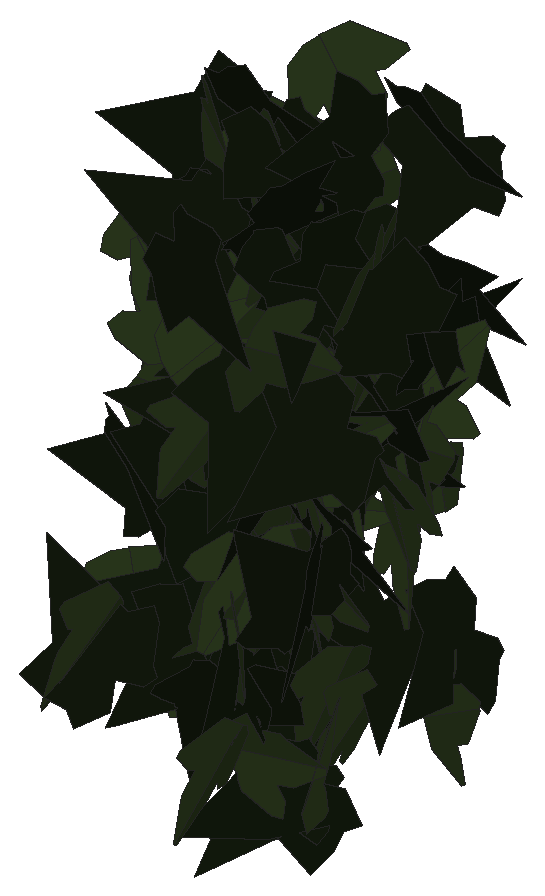
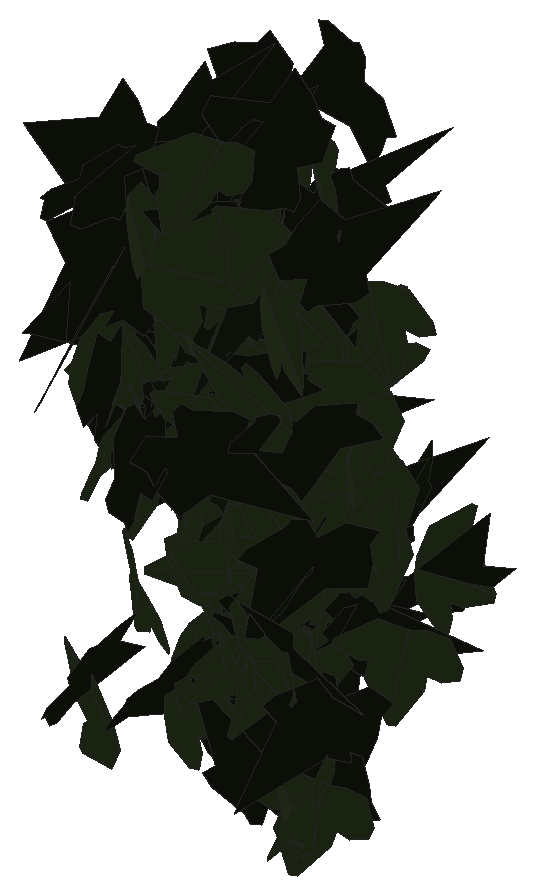
# SketchUp Ruby script. Lengths in inches.
U = 1.inch
M = Sketchup.active_model
def pt(a) = Geom::Point3d.new(a.map { |v| v * U })
def face(e, loops, mat)
  f = e.add_face(loops[0].map { |a| pt(a) })
  loops[1..].each { |l| e.add_face(l.map { |a| pt(a) }).erase! }
  f.material = f.back_material = mat if mat
  f
end
# faces: each face lists its corners as indices into pts; further lists are holes
def faces(e, pts, list, mat = nil) = list.each { |f| face(e, (f[0].is_a?(Array) ? f : [f]).map { |l| l.map { |i| pts[i] } }, mat) }
# xy, xz, yz: faces in a plane at the given z, y or x. An outline is a flat list of corners, or four numbers for a rectangle; further outlines are holes
def ring(l) = l.size == 4 ? [[l[0], l[1]], [l[2], l[1]], [l[2], l[3]], [l[0], l[3]]] : l.each_slice(2).to_a
def flat(e, list, mat, &to3) = list.each { |f| face(e, (f[0].is_a?(Array) ? f : [f]).map { |l| ring(l).map { |u, v| to3.(u, v) } }, mat) }
def xy(e, z, list, mat = nil) = flat(e, list, mat) { |x, y| [x, y, z] }
def xz(e, y, list, mat = nil) = flat(e, list, mat) { |x, z| [x, y, z] }
def yz(e, x, list, mat = nil) = flat(e, list, mat) { |y, z| [x, y, z] }
def lines(e, pts, list) = list.each { |a, b| e.add_line(pt(pts[a]), pt(pts[b])) }
# prism: a flat outline (further loops are holes) pulled along v
def prism(e, loops, v, mat = nil)
  f = face(e, loops, mat); d = Geom::Vector3d.new(v.map { |x| x * U })
  f.pushpull(f.normal.samedirection?(d) ? d.length : -d.length)
end
def box(e, o, s, mat = nil) = prism(e, [[o, [o[0] + s[0], o[1], o[2]], [o[0] + s[0], o[1] + s[1], o[2]], [o[0], o[1] + s[1], o[2]]]], [0, 0, s[2]], mat)
def at(x, y, z, deg = 0) = Geom::Transformation.translation(pt([x, y, z])) * Geom::Transformation.rotation(ORIGIN, Z_AXIS, deg.degrees)
def axes(o, x, y, z) = Geom::Transformation.new([*x, 0, *y, 0, *z, 0, *pt(o).to_a, 1])
def part(name) = M.definitions.add(name)
# library, detail: a bought-in or finely detailed component or shape, given as its bounding box
def library(name, o, s) = part(name).tap { |d| box(d.entities, o, s) }
def detail(e, o, s) = box(e.add_group.entities, o, s)
def put(e, d, t, mat = nil) = e.add_instance(d, t).tap { |i| i.material = mat if mat }
def group(e, t, mat = nil) = e.add_group.tap { |g| g.transformation = t; g.material = mat if mat }.entities
root = M.entities
M.materials.add("efeu1").color = [18, 25, 13]
M.materials.add("efeu2").color = [43, 57, 29]
c1 = part("ivyleaf_10")
p = [[0,0.5,-0.03],[-0.0625,2.02,-0.43],[-0.19,2.01,-0.46],[-0.54,1.05,-0.29],[-0.52,0.625,-0.18],[-0.83,0.76,-0.28],
  [-1.16,0.64,-0.33],[-1.15,0.33,-0.24],[-0.77,-0.39,0.02],[-0.3,-0.51,0.16],[0.04,-0.48,0.23],[-0.02,2.01,-0.4375],
  [-0.06,2.01,-0.43],[0.04,-0.49,0.23],[0.67,-0.49,0.14],[1.38,0.36,-0.2],[1.375,0.51,-0.24],[0.81,0.65,-0.19],
  [0.62,0.59,-0.15],[0.6,1.09,-0.28],[0.5,1.23,-0.31]]
faces(c1.entities,p,[[0,1,2,3,4,5,6,7,8,9,10],[11,12,0,13,14,15,16,17,18,19,20]],"efeu2")
c2 = part("ivyleaf_9")
p = [[1.54,2.16,1.25],[1.36,2.04,1.19],[-0.21,0.99,0.68],[-0.71,1.11,0.82],[-0.85,0.86,0.67],[-0.8,0.17,0.21],
  [-0.9,-0.01,0.1],[-0.67,-0.16,-0.02],[-0.08,-0.08,-0.05],[-0.03,-0.6,-0.4],[0.65,-0.88,-0.66],[0.83,-0.6,-0.49],
  [1.29,-0.42,-0.43],[1.8125,-0.07,-0.26],[1.21,0.44,0.15]]
faces(c2.entities,p,[[0,1,2,3,4,5,6,7,8,9,10,11,12,13,14]],"efeu1")
put(root,c1,axes([28.53,222.35,208.63],[0.41303,0.25945,0.10997],[0.09046,0.06274,-0.48773],[-0.26688,0.42279,0.00489]))
put(root,c2,axes([28.9,223.32,212.99],[-0.05885,-0.0343,0.49534],[-0.41168,-0.2755,-0.06799],[0.27759,-0.41584,0.00418]))
put(root,c1,axes([28.39,223.03,209.91],[-0.23609,-0.00713,0.4407],[0.44021,-0.02857,0.23536],[0.02183,0.49913,0.01977]))
put(root,c2,axes([28.59,223.36,208.42],[0.0425,-0.18384,-0.46303],[-0.03263,0.46269,-0.1867],[0.49712,0.04609,0.02733]))
put(root,c2,axes([28.59,223.66,210.3125],[-0.02142,-0.30956,-0.39207],[0.02032,0.39156,-0.31027],[0.49913,-0.02922,-0.00419]))
put(root,c1,axes([28.71,223.6,207.47],[-0.0357,0.46092,-0.19048],[0.01728,-0.18971,-0.46229],[-0.49842,-0.03959,-0.00238]))
put(root,c2,axes([28.98,222.45,209.85],[-0.08439,-0.03512,0.49157],[-0.37944,-0.31362,-0.08755],[0.31448,-0.38783,0.02628]))
put(root,c1,axes([28.68,222.5,209.8125],[-0.06336,-0.09851,-0.48609],[0.23876,0.42346,-0.11694],[0.43472,-0.24693,-0.00662]))
put(root,c1,axes([28.63,222.67,210.59],[-0.25398,-0.13068,-0.41039],[0.35505,0.20615,-0.28538],[0.24379,-0.43638,-0.01192]))
put(root,c1,axes([28.82,222.47,212.39],[0.4959,0.06356,-0.00651],[-0.00646,-0.00079,-0.49996],[-0.06356,0.49594,0.00004]))
put(root,c2,axes([28.6,222.36,209.89],[0.1419,-0.3425,0.3355],[0.12882,-0.30979,-0.37073],[0.46181,0.19164,0.00032]))
put(root,c1,axes([28.75,223.375,207.3125],[0.39362,0.258,0.16882],[0.14244,0.09063,-0.47063],[-0.27345,0.4186,-0.00215]))
put(root,c2,axes([28.84,223.625,211.5],[-0.19523,-0.4222,-0.18339],[0.08014,0.16498,-0.46514],[0.45328,-0.21101,0.00326]))
put(root,c1,axes([29.08,223.88,209.38],[0.0284,0.14804,0.47674],[-0.08611,-0.4689,0.15074],[0.49171,-0.09066,-0.00114]))
put(root,c1,axes([29.11,222.83,210.23],[-0.2734,-0.39024,0.15154],[-0.07857,-0.12995,-0.47638],[0.41119,-0.2843,0.00974]))
put(root,c1,axes([29.09,222.35,211.47],[0.21956,0.42607,0.14233],[-0.07184,-0.12307,0.47926],[0.44343,-0.23091,0.00717]))
put(root,c1,axes([28.76,222.89,210.82],[0.00696,-0.07393,0.49445],[0.38963,-0.30906,-0.0517],[0.31328,0.38603,0.05331]))
put(root,c2,axes([29.42,222.25,208.53],[-0.22412,-0.16527,-0.41528],[-0.29701,-0.29209,0.27653],[-0.334,0.37063,0.03275]))
put(root,c1,axes([29.04,221.26,208.84],[0.06989,-0.30517,0.38986],[0.06842,-0.38399,-0.31284],[0.49034,0.09708,-0.01191]))
put(root,c2,axes([29.26,221.14,208.36],[-0.3228,-0.36528,0.11122],[0.07397,0.08305,0.48747],[-0.3746,0.33117,0.00042]))
put(root,c2,axes([29.38,223.83,209.23],[-0.47607,0.06129,0.14],[-0.1384,0.02143,-0.47999],[-0.06483,-0.49577,-0.00344]))
put(root,c1,axes([28.78,222.67,211.36],[-0.26679,-0.05461,-0.41934],[0.41986,0.02495,-0.27037],[0.05045,-0.49638,0.03255]))
put(root,c2,axes([28.92,222.91,207.125],[-0.22378,0.19728,0.40126],[0.28261,-0.28531,0.29788],[0.34649,0.36011,0.01618]))
put(root,c2,axes([28.89,223.23,209.39],[0.08885,-0.43811,0.22397],[0.07088,-0.21382,-0.44638],[0.48691,0.11107,0.02411]))
put(root,c1,axes([29.51,223.5625,209.2],[-0.29558,0.01781,0.40288],[-0.40273,0.013,-0.29605],[-0.02102,-0.49951,0.00666]))
put(root,c1,axes([29.43,222.5,213.49],[0.03487,-0.05431,-0.49582],[-0.28405,0.40639,-0.06449],[0.41,0.28617,-0.00252]))
put(root,c1,axes([29.04,223.38,209.93],[-0.33146,-0.24207,0.28555],[0.22724,0.17298,0.41041],[-0.29749,0.40184,-0.00466]))
put(root,c1,axes([29,223.47,207],[0.10891,-0.26029,-0.41278],[0.18948,-0.3672,0.28154],[-0.44971,-0.21775,0.01866]))
put(root,c1,axes([29.2,223.52,212.58],[0.18011,-0.4462,0.13587],[0.05961,-0.12244,-0.4811],[0.46261,0.1895,0.00909]))
put(root,c2,axes([28.96,223.375,210],[0.40045,-0.29739,0.03462],[0.02954,-0.01829,-0.49879],[0.29794,0.40152,0.00292]))
put(root,c1,axes([29.04,223.83,211.61],[0.1946,-0.11111,-0.44698],[0.43679,-0.1094,0.21736],[-0.1461,-0.47507,0.05448]))
put(root,c2,axes([29.5,222.26,208.32],[-0.20028,-0.33528,0.31221],[-0.13768,-0.28094,-0.39002],[0.43696,-0.2422,0.0202]))
put(root,c2,axes([29.63,222.38,213.13],[0.16965,0.3322,-0.33296],[-0.15665,-0.29384,-0.37299],[-0.44349,0.23087,0.00438]))
put(root,c2,axes([29.87,222.57,210.72],[-0.22977,-0.01906,0.44367],[-0.42908,-0.11919,-0.22734],[0.11442,-0.48521,0.03842]))
put(root,c1,axes([29.51,223.08,208.65],[-0.09599,-0.36957,-0.32281],[0.10935,0.30455,-0.38117],[0.47836,-0.14378,0.02236]))
put(root,c1,axes([29.28,223.35,213.18],[0.35513,0.15313,0.31691],[0.27792,0.15425,-0.38596],[-0.21598,0.45029,0.02445]))
put(root,c2,axes([29.77,223.15,208.91],[-0.20539,-0.45247,0.05557],[0.02282,0.05066,0.4969],[-0.45529,0.20666,-0.00016]))
put(root,c2,axes([29.86,223.25,211.42],[-0.37609,-0.15108,0.2928],[-0.26238,-0.13143,-0.40483],[0.19929,-0.45815,0.01958]))
put(root,c1,axes([29.62,222.43,208.1875],[-0.21941,-0.42087,-0.15726],[-0.07553,-0.13797,0.47461],[-0.44289,0.23203,-0.00304]))
put(root,c2,axes([29.84,221.98,212.85],[-0.14868,-0.45257,-0.1519],[-0.04712,-0.14441,0.47637],[-0.47505,0.15596,0.0003]))
put(root,c1,axes([29.39,223.08,207.32],[-0.10173,0.06211,-0.48559],[0.26917,-0.40716,-0.10847],[-0.4089,-0.28348,0.04941]))
put(root,c2,axes([29.45,222.46,209.73],[-0.03037,-0.18216,-0.46464],[0.09404,0.45508,-0.18456],[0.49014,-0.0986,0.00661]))
put(root,c2,axes([29.45,223.36,207.04],[-0.24696,0.15292,0.40697],[0.33971,-0.2242,0.2904],[0.2713,0.41994,0.00684]))
put(root,c1,axes([29.5,223.21,208.83],[-0.21458,-0.22682,-0.39052],[0.2738,0.27851,-0.3122],[0.35915,-0.34783,0.00469]))
put(root,c2,axes([29.96,223.98,211.08],[-0.00622,-0.02552,-0.49931],[-0.28381,-0.41091,0.02454],[-0.4116,0.28372,-0.00938]))
put(root,c1,axes([29.82,222.05,210.96],[-0.15263,-0.38626,0.2784],[-0.10006,-0.25981,-0.41532],[0.4655,-0.18249,0.00201]))
put(root,c2,axes([29.72,223.16,208.4],[-0.16359,-0.35359,0.31339],[-0.10166,-0.29754,-0.38876],[0.46141,-0.19091,0.02545]))
put(root,c1,axes([29.35,222.58,211.75],[0.19852,-0.09898,-0.4481],[0.43122,-0.12677,0.21904],[-0.15697,-0.47343,0.03503]))
put(root,c2,axes([29.64,223.15,212.63],[0.42868,-0.14007,-0.21591],[-0.19868,0.08651,-0.4506],[0.16359,0.47212,0.01851]))
put(root,c1,axes([29.47,223.39,208.5625],[-0.21608,-0.02939,0.44994],[0.45014,0.01494,0.21715],[-0.02621,0.49891,0.02]))
put(root,c1,axes([29.51,222.04,211.44],[0.34751,0.03758,-0.35753],[0.35077,0.07348,0.34866],[0.07875,-0.49314,0.0247]))
put(root,c1,axes([29.9,222.79,212.26],[-0.31127,0.36037,0.15245],[0.09972,-0.11532,0.47619],[0.37837,0.32685,-0.00008]))
put(root,c1,axes([29.64,222.79,210.96],[-0.27001,-0.10107,0.40851],[0.38167,0.14563,0.2883],[-0.17726,0.46752,-0.0015]))
put(root,c1,axes([30.15,223.9,212.82],[-0.05548,-0.14035,0.47668],[-0.21545,-0.42542,-0.15034],[0.44777,-0.22209,-0.01328]))
put(root,c1,axes([29.99,222.97,209.84],[0.06967,-0.49414,-0.03118],[-0.00418,0.0309,-0.49903],[0.4951,0.0698,0.00017]))
put(root,c2,axes([30.11,221.84,208.27],[0.17058,0.33736,-0.32725],[-0.13902,-0.29634,-0.37796],[-0.44897,0.21993,-0.0073]))
put(root,c2,axes([29.58,222.78,213.72],[0.18882,-0.13886,0.44166],[0.37339,-0.23633,-0.23393],[0.27373,0.41817,0.01445]))
put(root,c1,axes([29.73,223.2,209.39],[-0.01836,-0.00413,0.49965],[0.33582,0.37011,0.0154],[-0.36998,0.33615,-0.01082]))
put(root,c1,axes([29.88,223.66,214.0625],[0.24573,0.38366,0.20596],[0.11046,0.17384,-0.45561],[-0.42121,0.26941,0.00067]))
put(root,c1,axes([30.08,223.32,211.49],[0.30746,0.358,-0.16524],[-0.1189,-0.1156,-0.4717],[-0.37594,0.32935,0.01405]))
put(root,c1,axes([30,223.2,209.23],[-0.02166,0.22627,-0.44534],[0.0489,-0.44266,-0.22729],[-0.49713,-0.0534,-0.00296]))
put(root,c1,axes([30.06,222.95,209.15],[-0.27796,0.36649,-0.19602],[0.12211,-0.15339,-0.45995],[-0.39727,-0.30357,-0.00423]))
put(root,c1,axes([29.88,223.56,211.02],[0.29921,0.17766,0.35904],[0.30459,0.19019,-0.34793],[-0.2602,0.42693,0.00559]))
put(root,c1,axes([30.23,222.6,212.7],[-0.11236,-0.38328,-0.30079],[0.09601,0.28521,-0.3993],[0.47766,-0.14749,0.0095]))
put(root,c2,axes([30.1,222.55,213.86],[0.10629,-0.44883,-0.19302],[-0.03713,0.18955,-0.46119],[0.48716,0.11237,0.00696]))
put(root,c2,axes([30.47,222.48,207.22],[-0.4813,-0.13394,0.0203],[-0.01777,-0.01187,-0.49954],[0.1343,-0.48158,0.00666]))
put(root,c1,axes([29.93,222.66,213.38],[-0.07405,-0.00916,0.4944],[0.48774,-0.08363,0.07151],[0.08138,0.49287,0.02132]))
put(root,c1,axes([30.32,222.29,209.21],[0.05219,-0.47919,0.13287],[0.01929,-0.13154,-0.482],[0.49689,0.05544,0.00476]))
put(root,c1,axes([30.03,223.15,209.58],[0.39852,-0.01726,0.30146],[0.30082,-0.0207,-0.39885],[0.02625,0.49927,-0.00612]))
put(root,c1,axes([30.41,221.84,209.58],[0.45072,0.08584,-0.1987],[-0.19574,-0.03429,-0.45882],[-0.0924,0.49138,0.00269]))
put(root,c2,axes([30.19,222.09,208.5625],[0.13456,-0.1799,-0.44669],[0.33349,-0.29976,0.22119],[-0.34738,-0.35746,0.03931]))
put(root,c1,axes([30.6,222.81,209.5],[-0.0107,-0.04436,0.49791],[-0.21609,-0.44868,-0.04462],[0.45077,-0.21614,-0.00957]))
put(root,c1,axes([30.28,223.28,209.16],[0.05391,-0.42935,-0.2505],[0.0899,-0.23939,0.42966],[-0.48889,-0.09136,0.05138]))
put(root,c2,axes([30.72,222.26,207.21],[-0.00946,-0.02614,-0.49923],[-0.28126,-0.41251,0.02692],[-0.41328,0.28133,-0.0069]))
put(root,c1,axes([30.68,223.15,210.94],[0.27821,-0.18465,-0.37217],[-0.31072,0.20484,-0.3339],[0.27577,0.41707,-0.00077]))
put(root,c2,axes([30.49,221.97,211.48],[-0.30326,-0.39748,-0.00696],[0.00421,0.00554,-0.49995],[0.39751,-0.30329,-0.00002]))
put(root,c1,axes([30.55,222.31,212.32],[-0.17967,-0.4662,-0.01931],[0.00679,0.01808,-0.49963],[0.46655,-0.1798,-0.00016]))
put(root,c2,axes([30.56,222.97,209.54],[0.1917,-0.44754,0.11386],[-0.04035,0.10658,0.48684],[-0.46003,-0.19584,0.00475]))
put(root,c2,axes([30.35,223.85,208.28],[0.00971,-0.49684,0.05531],[0.00627,-0.0552,-0.4969],[0.49987,0.01034,0.00516]))
put(root,c1,axes([30.24,221.8,208.67],[-0.03668,0.03164,0.49765],[0.40513,-0.28904,0.04824],[0.29073,0.40676,-0.00443]))
put(root,c1,axes([30.59,222.89,208.13],[-0.03118,-0.46582,0.179],[-0.00346,-0.17915,-0.46679],[0.49901,-0.03035,0.00795]))
put(root,c1,axes([30.375,223.45,211.91],[0.34671,-0.29606,-0.20528],[0.1551,-0.13448,0.45592],[-0.32517,-0.37982,-0.00141]))
put(root,c1,axes([30.24,221.95,207.48],[-0.13331,-0.04363,0.47992],[0.47615,0.06476,0.13815],[-0.07421,0.49386,0.02428]))
put(root,c2,axes([30.63,223.0625,212.87],[-0.3354,-0.35403,-0.11031],[0.07744,0.07858,-0.48768],[0.36264,-0.34422,0.00212]))
put(root,c1,axes([30.62,223.14,207.6],[0.08251,-0.25721,0.42076],[0.11523,-0.40474,-0.27001],[0.47949,0.14153,-0.00751]))
put(root,c2,axes([30.33,220.79,213.47],[-0.00168,-0.08886,-0.49204],[0.47854,0.1423,-0.02733],[0.14489,-0.47102,0.08456]))
put(root,c1,axes([30.46,222.1,209.18],[-0.30044,0.10956,0.38436],[0.35953,-0.13595,0.31978],[0.17457,0.46853,0.00291]))
put(root,c1,axes([30.74,220.99,208.17],[0.06593,-0.40116,0.29108],[0.0456,-0.28749,-0.40654],[0.49353,0.08015,-0.00132]))
put(root,c2,axes([30.53,223.04,210.38],[0.09739,-0.08149,-0.48361],[0.3791,-0.30029,0.12694],[-0.31113,-0.39139,0.0033]))
put(root,c1,axes([30.51,223.91,209.23],[0.33564,-0.16232,0.33316],[0.29744,-0.15014,-0.37281],[0.22107,0.44846,-0.00423]))
put(root,c2,axes([30.6875,221.58,213.54],[0.20954,0.33234,0.30926],[0.15527,0.26761,-0.39278],[-0.4266,0.26065,0.00895]))
put(root,c2,axes([30.9,221.65,210.97],[-0.21957,0.36267,-0.26506],[0.1394,-0.22545,-0.42395],[-0.42703,-0.26008,-0.00211]))
put(root,c2,axes([30.83,223,213.67],[-0.09275,-0.11655,0.4773],[-0.22981,-0.41903,-0.14698],[0.43426,-0.24664,0.02416]))
put(root,c1,axes([30.87,223.53,212.97],[0.19466,-0.45908,-0.03671],[-0.01273,0.03447,-0.49865],[0.46037,0.19507,0.00173]))
put(root,c2,axes([30.63,223.09,211.39],[0.38513,-0.24445,-0.20475],[0.18246,-0.09436,0.45585],[-0.2615,-0.42584,0.01652]))
put(root,c2,axes([30.57,223.89,210.32],[0.01533,-0.12557,0.48373],[0.20756,-0.43865,-0.12044],[0.45463,0.2045,0.03868]))
put(root,c1,axes([30.93,222.82,211.67],[0.03047,-0.49551,0.05951],[0.00146,-0.05953,-0.49644],[0.49907,0.03043,-0.00218]))
put(root,c1,axes([30.97,221.94,210.93],[-0.14757,0.47766,0.00789],[-0.0034,0.00721,-0.49994],[-0.47772,-0.1476,0.00112]))
put(root,c2,axes([31.01,221.84,213.08],[0.00357,-0.04239,-0.49819],[-0.18915,0.46106,-0.04059],[0.46283,0.18875,-0.01275]))
put(root,c2,axes([30.99,223.97,211.09],[0.01493,0.03016,0.49887],[-0.15949,-0.47271,0.03335],[0.47365,-0.16012,-0.00449]))
put(root,c1,axes([30.95,222.07,207.29],[0.31032,-0.38898,-0.04897],[0.03191,-0.03719,0.49759],[-0.39075,-0.31195,0.00174]))
put(root,c1,axes([30.9,221.92,210.83],[-0.05954,-0.15567,0.47141],[0.13862,0.45069,0.16633],[-0.4767,0.1505,-0.01051]))
put(root,c2,axes([30.84,222.13,210.25],[0.49815,-0.03061,-0.03012],[-0.03006,0.00183,-0.49909],[0.03067,0.49906,-0.00002]))
put(root,c2,axes([30.87,221.87,212.99],[0.04763,-0.47149,0.15947],[0.03452,-0.15668,-0.47356],[0.49653,0.05612,0.01763]))
put(root,c1,axes([30.71,222.28,209.48],[-0.00042,-0.11261,0.48715],[0.49625,-0.05965,-0.01336],[0.06112,0.48349,0.11181]))
put(root,c2,axes([31.16,221.64,209.49],[0.129,0.15876,0.45624],[-0.35504,-0.28906,0.20097],[0.32757,-0.37582,0.03816]))
put(root,c1,axes([31.15,223.01,210.26],[-0.47635,0.14898,0.02998],[-0.02897,0.00781,-0.4991],[-0.14918,-0.47723,0.0012]))
put(root,c2,axes([30.875,222.5,210.65],[0.12612,0.459,-0.15302],[0.03939,0.14786,0.47601],[0.48222,-0.13213,0.00114]))
put(root,c2,axes([31.1,222.92,210.33],[-0.40754,-0.03861,0.28709],[0.28936,-0.07734,0.40036],[0.01349,0.49247,0.08538]))
put(root,c1,axes([31.11,223.87,211.57],[-0.02599,-0.37272,0.33227],[0.09085,-0.3307,-0.36385],[0.49099,0.04145,0.08491]))
put(root,c2,axes([31.12,224.2,208.12],[-0.09904,-0.36416,0.32799],[-0.08791,-0.316,-0.37738],[0.48214,-0.13242,-0.00143]))
put(root,c2,axes([31.1875,223.96,213.51],[-0.20765,-0.43369,0.13709],[-0.05053,-0.12777,-0.48075],[0.45202,-0.21351,0.00923]))
put(root,c2,axes([30.98,223.1,210.53],[0.49615,-0.03977,-0.04744],[0.04741,-0.00237,0.49774],[-0.03982,-0.49841,0.00142]))
put(root,c1,axes([31.29,222.46,212.86],[0.11949,-0.45837,-0.16004],[-0.01761,0.16062,-0.47317],[0.48519,0.11872,0.02224]))
put(root,c1,axes([31.33,223.42,210.13],[-0.08143,0.47254,-0.14168],[-0.04124,0.13657,0.47921],[0.4916,0.08974,0.01674]))
put(root,c1,axes([31.15,221.04,212.57],[-0.14512,-0.24384,-0.41168],[0.2091,0.35463,-0.28375],[0.43037,-0.25452,-0.00095]))
put(root,c2,axes([30.87,223.81,213.62],[0.24556,-0.21367,0.37953],[0.30664,-0.22461,-0.32485],[0.30931,0.3923,0.02073]))
put(root,c2,axes([31.12,223.33,212.41],[0.46877,0.16233,0.06248],[0.05948,0.01918,-0.49608],[-0.16345,0.47253,-0.00133]))
put(root,c2,axes([31.72,222.4,212.36],[-0.06529,0.02615,0.49503],[-0.49535,-0.02267,-0.06414],[0.01909,-0.4988,0.02886]))
put(root,c1,axes([31.1,223.76,207.44],[0.18662,-0.14451,-0.44078],[0.33321,-0.28877,0.23575],[-0.32271,-0.38174,-0.01148]))
put(root,c2,axes([31.33,223.45,212.11],[0.30817,-0.23121,-0.3187],[-0.23044,0.22225,-0.38406],[0.31926,0.3836,0.03042]))
put(root,c2,axes([31.32,221.65,210.09],[-0.12708,-0.00206,-0.48358],[0.42338,-0.24207,-0.11023],[-0.23366,-0.43749,0.06327]))
put(root,c1,axes([31.21,223.26,211.14],[0.39657,-0.04606,-0.30101],[0.30448,0.06801,0.39073],[0.00495,-0.49321,0.08199]))
put(root,c2,axes([31.44,223.02,211.72],[0.11184,0.19149,0.44813],[0.21237,0.39468,-0.22165],[-0.43863,0.23991,0.00694]))
put(root,c2,axes([31.62,221.64,211.59],[-0.28558,-0.3166,0.26117],[-0.14926,-0.21627,-0.42538],[0.38232,-0.32093,0.02901]))
put(root,c1,axes([31.21,223.22,210.62],[0.11106,-0.1009,-0.47695],[0.35875,-0.3143,0.15003],[-0.33009,-0.37554,0.00259]))
